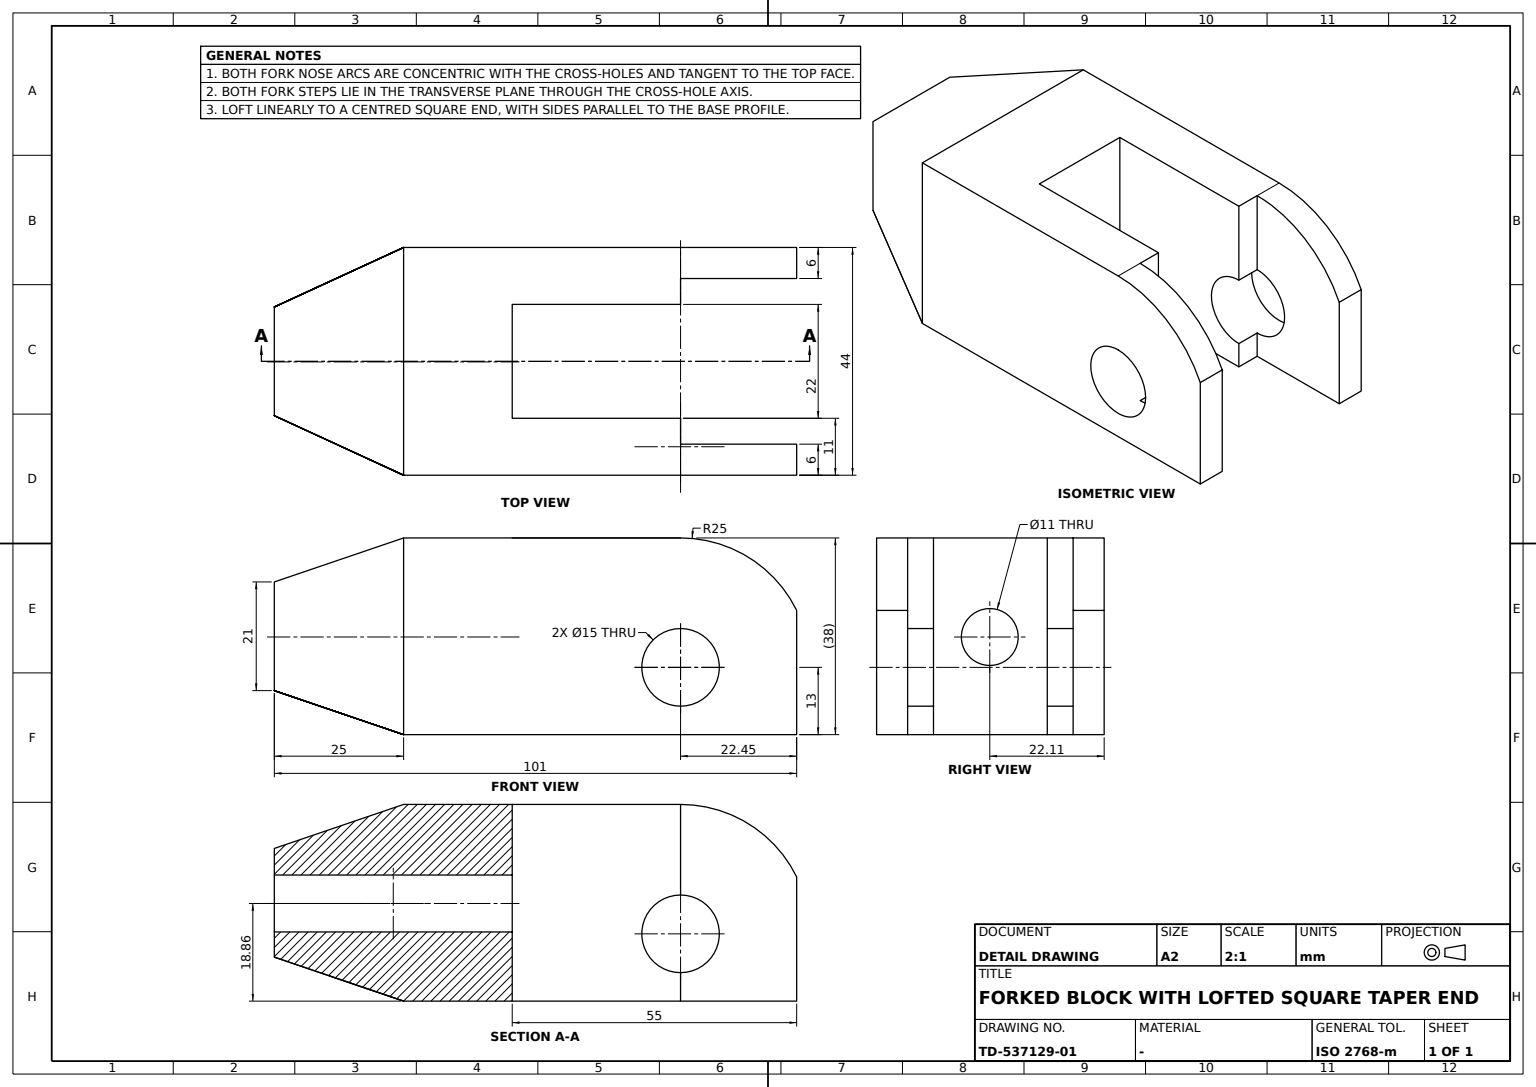
ISO-10303-21;
HEADER;
FILE_DESCRIPTION((''),'2;1');
FILE_NAME('','',(''),(''),'','','');
FILE_SCHEMA(('AUTOMOTIVE_DESIGN'));
ENDSEC;
DATA;
#1=APPLICATION_CONTEXT('');
#2=PRODUCT_CONTEXT('',#1,'mechanical');
#3=PRODUCT('','','',(#2));
#4=PRODUCT_DEFINITION_FORMATION('','',#3);
#5=PRODUCT_DEFINITION_CONTEXT('',#1,'design');
#6=PRODUCT_DEFINITION('','',#4,#5);
#7=PRODUCT_DEFINITION_SHAPE('','',#6);
#8=(LENGTH_UNIT()NAMED_UNIT(*)SI_UNIT(.MILLI.,.METRE.));
#9=(NAMED_UNIT(*)PLANE_ANGLE_UNIT()SI_UNIT($,.RADIAN.));
#10=(NAMED_UNIT(*)SI_UNIT($,.STERADIAN.)SOLID_ANGLE_UNIT());
#11=UNCERTAINTY_MEASURE_WITH_UNIT(LENGTH_MEASURE(1.E-05),#8,'distance_accuracy_value','');
#12=(GEOMETRIC_REPRESENTATION_CONTEXT(3)GLOBAL_UNCERTAINTY_ASSIGNED_CONTEXT((#11))GLOBAL_UNIT_ASSIGNED_CONTEXT((#8,#9,#10))REPRESENTATION_CONTEXT('',''));
#13=CARTESIAN_POINT('',(22.449944,16.,5.5));
#14=VERTEX_POINT('',#13);
#15=CARTESIAN_POINT('',(22.449944,22.,5.5));
#16=VERTEX_POINT('',#15);
#17=CARTESIAN_POINT('',(22.449944,-22.,5.5));
#18=DIRECTION('',(0.,1.,0.));
#19=VECTOR('',#18,1000.);
#20=LINE('',#17,#19);
#21=EDGE_CURVE('',#14,#16,#20,.T.);
#22=ORIENTED_EDGE('',*,*,#21,.T.);
#23=CARTESIAN_POINT('',(22.449944,22.,20.5));
#24=VERTEX_POINT('',#23);
#25=CARTESIAN_POINT('',(22.449944,22.,13.));
#26=DIRECTION('',(0.,-1.,0.));
#27=DIRECTION('',(1.,0.,0.));
#28=AXIS2_PLACEMENT_3D('',#25,#26,#27);
#29=CIRCLE('',#28,7.5);
#30=EDGE_CURVE('',#24,#16,#29,.T.);
#31=ORIENTED_EDGE('',*,*,#30,.F.);
#32=CARTESIAN_POINT('',(22.449944,16.,20.5));
#33=VERTEX_POINT('',#32);
#34=CARTESIAN_POINT('',(22.449944,-22.,20.5));
#35=LINE('',#34,#19);
#36=EDGE_CURVE('',#33,#24,#35,.T.);
#37=ORIENTED_EDGE('',*,*,#36,.F.);
#38=CARTESIAN_POINT('',(22.449944,16.,13.));
#39=DIRECTION('',(0.,0.,-1.));
#40=AXIS2_PLACEMENT_3D('',#38,#26,#39);
#41=CIRCLE('',#40,7.5);
#42=EDGE_CURVE('',#33,#14,#41,.T.);
#43=ORIENTED_EDGE('',*,*,#42,.T.);
#44=EDGE_LOOP('',(#22,#31,#37,#43));
#45=FACE_OUTER_BOUND('',#44,.T.);
#46=CARTESIAN_POINT('',(22.449944,-22.,13.));
#47=DIRECTION('',(0.,0.,1.));
#48=AXIS2_PLACEMENT_3D('',#46,#18,#47);
#49=CYLINDRICAL_SURFACE('',#48,7.5);
#50=ADVANCED_FACE('',(#45),#49,.F.);
#51=CARTESIAN_POINT('',(101.,10.495948,8.504359));
#52=VERTEX_POINT('',#51);
#53=CARTESIAN_POINT('',(76.,21.993633,0.005916));
#54=VERTEX_POINT('',#53);
#55=CARTESIAN_POINT('',(92.666667,14.327802,5.672203));
#56=CARTESIAN_POINT('',(84.333333,18.159656,2.840046));
#57=B_SPLINE_CURVE_WITH_KNOTS('',3,(#51,#55,#56,#53),.UNSPECIFIED.,.F.,.F.,(4,4),(0.,1.),.UNSPECIFIED.);
#58=EDGE_CURVE('',#52,#54,#57,.T.);
#59=ORIENTED_EDGE('',*,*,#58,.T.);
#60=CARTESIAN_POINT('',(76.,21.998212,2.362252));
#61=VERTEX_POINT('',#60);
#62=CARTESIAN_POINT('',(76.,22.005328,0.020728));
#63=CARTESIAN_POINT('',(76.,21.997336,0.079513));
#64=CARTESIAN_POINT('',(76.,22.001332,0.178516));
#65=CARTESIAN_POINT('',(76.,21.999112,0.360332));
#66=CARTESIAN_POINT('',(76.,22.000592,0.718464));
#67=CARTESIAN_POINT('',(76.,21.999652,1.404027));
#68=CARTESIAN_POINT('',(76.,21.999859,1.985808));
#69=B_SPLINE_CURVE_WITH_KNOTS('',3,(#53,#62,#63,#64,#65,#66,#67,#68,#60),.UNSPECIFIED.,.F.,.F.,(4,1,1,1,1,1,4),(0.,0.000976562,0.001953125,0.00390625,0.0078125,0.015625,0.02994468),.UNSPECIFIED.);
#70=EDGE_CURVE('',#54,#61,#69,.T.);
#71=ORIENTED_EDGE('',*,*,#70,.T.);
#72=CARTESIAN_POINT('',(76.,21.992469,37.990831));
#73=VERTEX_POINT('',#72);
#74=CARTESIAN_POINT('',(76.,21.999974,2.396567));
#75=CARTESIAN_POINT('',(76.,22.000206,3.252405));
#76=CARTESIAN_POINT('',(76.,21.999825,5.752273));
#77=CARTESIAN_POINT('',(76.,22.000117,11.504111));
#78=CARTESIAN_POINT('',(76.,21.999961,19.721555));
#79=CARTESIAN_POINT('',(76.,22.,27.938819));
#80=CARTESIAN_POINT('',(76.,22.,33.690928));
#81=CARTESIAN_POINT('',(76.,22.,36.361551));
#82=CARTESIAN_POINT('',(76.,22.,37.491429));
#83=CARTESIAN_POINT('',(76.,22.,37.812418));
#84=CARTESIAN_POINT('',(76.,22.,37.940813));
#85=CARTESIAN_POINT('',(76.,22.002328,37.971865));
#86=CARTESIAN_POINT('',(76.,21.997745,37.986565));
#87=CARTESIAN_POINT('',(76.,21.993856,37.989071));
#88=B_SPLINE_CURVE_WITH_KNOTS('',3,(#60,#74,#75,#76,#77,#78,#79,#80,#81,#82,#83,#84,#85,#86,#87,#72),.UNSPECIFIED.,.F.,.F.,(4,1,1,1,1,1,1,1,1,1,1,1,1,4),(0.02994468,0.03125,0.0625,0.125,0.25,0.375,0.4375,0.46875,0.4765625,0.48046875,0.480957031,0.481445312,0.481567383,0.481678034),.UNSPECIFIED.);
#89=EDGE_CURVE('',#61,#73,#88,.T.);
#90=ORIENTED_EDGE('',*,*,#89,.T.);
#91=CARTESIAN_POINT('',(76.,-22.,38.));
#92=VERTEX_POINT('',#91);
#93=CARTESIAN_POINT('',(76.,-7.333333,38.));
#94=CARTESIAN_POINT('',(76.,7.333333,38.));
#95=B_SPLINE_CURVE_WITH_KNOTS('',3,(#91,#93,#94,#72),.UNSPECIFIED.,.F.,.F.,(4,4),(0.,1.),.UNSPECIFIED.);
#96=EDGE_CURVE('',#92,#73,#95,.T.);
#97=ORIENTED_EDGE('',*,*,#96,.F.);
#98=CARTESIAN_POINT('',(101.,-10.5,29.5));
#99=VERTEX_POINT('',#98);
#100=CARTESIAN_POINT('',(84.333333,-18.166667,35.166667));
#101=CARTESIAN_POINT('',(92.666667,-14.333333,32.333333));
#102=B_SPLINE_CURVE_WITH_KNOTS('',3,(#91,#100,#101,#98),.UNSPECIFIED.,.F.,.F.,(4,4),(0.,1.),.UNSPECIFIED.);
#103=EDGE_CURVE('',#92,#99,#102,.T.);
#104=ORIENTED_EDGE('',*,*,#103,.T.);
#105=CARTESIAN_POINT('',(101.,10.502543,8.511455));
#106=CARTESIAN_POINT('',(101.,10.498729,8.543941));
#107=CARTESIAN_POINT('',(101.,10.500636,8.598653));
#108=CARTESIAN_POINT('',(101.,10.499576,8.699131));
#109=CARTESIAN_POINT('',(101.,10.500283,8.897046));
#110=CARTESIAN_POINT('',(101.,10.499812,9.294902));
#111=CARTESIAN_POINT('',(101.,10.500126,10.089264));
#112=CARTESIAN_POINT('',(101.,10.499916,11.678888));
#113=CARTESIAN_POINT('',(101.,10.500056,14.857535));
#114=CARTESIAN_POINT('',(101.,10.501476,19.400362));
#115=CARTESIAN_POINT('',(101.,10.495516,23.935049));
#116=CARTESIAN_POINT('',(101.,10.506725,27.125907));
#117=CARTESIAN_POINT('',(101.,10.491593,28.585496));
#118=CARTESIAN_POINT('',(101.,10.506305,29.225732));
#119=CARTESIAN_POINT('',(101.,10.492664,29.388443));
#120=CARTESIAN_POINT('',(101.,10.503941,29.471531));
#121=CARTESIAN_POINT('',(101.,10.502736,29.4862));
#122=CARTESIAN_POINT('',(101.,10.498467,29.49225));
#123=CARTESIAN_POINT('',(101.,10.494805,29.495405));
#124=CARTESIAN_POINT('',(101.,10.486541,29.498931));
#125=CARTESIAN_POINT('',(101.,10.464878,29.500457));
#126=CARTESIAN_POINT('',(101.,10.432319,29.500903));
#127=CARTESIAN_POINT('',(101.,10.398751,29.500263));
#128=CARTESIAN_POINT('',(101.,10.278255,29.498336));
#129=CARTESIAN_POINT('',(101.,10.067183,29.498289));
#130=CARTESIAN_POINT('',(101.,9.023461,29.503487));
#131=CARTESIAN_POINT('',(101.,7.226471,29.5));
#132=CARTESIAN_POINT('',(101.,3.85,29.5));
#133=CARTESIAN_POINT('',(101.,-2.058824,29.5));
#134=CARTESIAN_POINT('',(101.,-7.123529,29.5));
#135=B_SPLINE_CURVE_WITH_KNOTS('',3,(#51,#105,#106,#107,#108,#109,#110,#111,#112,#113,#114,#115,#116,#117,#118,#119,#120,#121,#122,#123,#124,#125,#126,#127,#128,#129,#130,#131,#132,#133,#134,#98),.UNSPECIFIED.,.F.,.F.,(4,1,1,1,1,1,1,1,1,1,1,1,1,1,1,1,1,1,1,1,1,1,1,1,1,1,1,1,1,4),(0.,0.000976562,0.001953125,0.00390625,0.0078125,0.015625,0.03125,0.0625,0.125,0.25,0.375,0.4375,0.46875,0.4765625,0.48046875,0.480957031,0.481445312,0.481567383,0.481689453,0.481933594,0.482421875,0.483398438,0.484375,0.484863281,0.4921875,0.5,0.5625,0.625,0.75,1.),.UNSPECIFIED.);
#136=EDGE_CURVE('',#52,#99,#135,.T.);
#137=ORIENTED_EDGE('',*,*,#136,.F.);
#138=EDGE_LOOP('',(#59,#71,#90,#97,#104,#137));
#139=FACE_OUTER_BOUND('',#138,.T.);
#140=CARTESIAN_POINT('',(76.,21.991511,0.007889));
#141=CARTESIAN_POINT('',(92.666667,14.336805,5.681213));
#142=CARTESIAN_POINT('',(84.333333,18.171066,2.85097));
#143=CARTESIAN_POINT('',(92.666667,14.331598,5.722465));
#144=CARTESIAN_POINT('',(84.333333,18.164467,2.900989));
#145=CARTESIAN_POINT('',(92.666667,14.334201,5.791941));
#146=CARTESIAN_POINT('',(84.333333,18.167767,2.985228));
#147=CARTESIAN_POINT('',(92.666667,14.332755,5.919531));
#148=CARTESIAN_POINT('',(84.333333,18.165933,3.139932));
#149=CARTESIAN_POINT('',(92.666667,14.333719,6.170852));
#150=CARTESIAN_POINT('',(84.333333,18.167156,3.444658));
#151=CARTESIAN_POINT('',(92.666667,14.333076,6.676066));
#152=CARTESIAN_POINT('',(84.333333,18.166341,4.05723));
#153=CARTESIAN_POINT('',(76.,21.999605,1.438394));
#154=CARTESIAN_POINT('',(92.666667,14.333505,7.684779));
#155=CARTESIAN_POINT('',(84.333333,18.166884,5.280295));
#156=CARTESIAN_POINT('',(76.,22.000263,2.87581));
#157=CARTESIAN_POINT('',(92.666667,14.333219,9.703349));
#158=CARTESIAN_POINT('',(84.333333,18.166522,7.727811));
#159=CARTESIAN_POINT('',(92.666667,14.33341,13.739727));
#160=CARTESIAN_POINT('',(84.333333,18.166763,12.621919));
#161=CARTESIAN_POINT('',(92.666667,14.334304,19.507427));
#162=CARTESIAN_POINT('',(84.333333,18.167133,19.614491));
#163=CARTESIAN_POINT('',(92.666667,14.330344,25.269639));
#164=CARTESIAN_POINT('',(84.333333,18.165172,26.604229));
#165=CARTESIAN_POINT('',(92.666667,14.337817,29.314248));
#166=CARTESIAN_POINT('',(84.333333,18.168908,31.502588));
#167=CARTESIAN_POINT('',(92.666667,14.327729,31.177514));
#168=CARTESIAN_POINT('',(84.333333,18.163864,33.769532));
#169=CARTESIAN_POINT('',(92.666667,14.337537,31.980964));
#170=CARTESIAN_POINT('',(84.333333,18.168768,34.736197));
#171=CARTESIAN_POINT('',(92.666667,14.328443,32.196435));
#172=CARTESIAN_POINT('',(84.333333,18.164221,35.004426));
#173=CARTESIAN_POINT('',(92.666667,14.33596,32.294625));
#174=CARTESIAN_POINT('',(84.333333,18.16798,35.117719));
#175=CARTESIAN_POINT('',(92.666667,14.335933,32.314755));
#176=CARTESIAN_POINT('',(84.333333,18.169131,35.14331));
#177=CARTESIAN_POINT('',(92.666667,14.331535,32.323766));
#178=CARTESIAN_POINT('',(84.333333,18.164604,35.155282));
#179=CARTESIAN_POINT('',(76.,21.997672,37.986798));
#180=CARTESIAN_POINT('',(92.666667,14.326291,32.327545));
#181=CARTESIAN_POINT('',(84.333333,18.157778,35.159685));
#182=CARTESIAN_POINT('',(76.,21.989264,37.991825));
#183=CARTESIAN_POINT('',(92.666667,14.317459,32.334298));
#184=CARTESIAN_POINT('',(84.333333,18.148378,35.169664));
#185=CARTESIAN_POINT('',(76.,21.979296,38.005031));
#186=CARTESIAN_POINT('',(92.666667,14.284217,32.332825));
#187=CARTESIAN_POINT('',(84.333333,18.103556,35.165193));
#188=CARTESIAN_POINT('',(76.,21.922896,37.997561));
#189=CARTESIAN_POINT('',(92.666667,14.239395,32.333041));
#190=CARTESIAN_POINT('',(84.333333,18.046471,35.165179));
#191=CARTESIAN_POINT('',(76.,21.853546,37.997317));
#192=CARTESIAN_POINT('',(92.666667,14.19507,32.333621));
#193=CARTESIAN_POINT('',(84.333333,17.991389,35.166978));
#194=CARTESIAN_POINT('',(76.,21.787708,38.000335));
#195=CARTESIAN_POINT('',(92.666667,14.031715,32.332224));
#196=CARTESIAN_POINT('',(84.333333,17.785174,35.166112));
#197=CARTESIAN_POINT('',(76.,21.538634,38.));
#198=CARTESIAN_POINT('',(92.666667,13.743614,32.332193));
#199=CARTESIAN_POINT('',(84.333333,17.420045,35.166096));
#200=CARTESIAN_POINT('',(76.,21.096477,38.));
#201=CARTESIAN_POINT('',(92.666667,12.315477,32.335658));
#202=CARTESIAN_POINT('',(84.333333,15.607494,35.167829));
#203=CARTESIAN_POINT('',(76.,18.89951,38.));
#204=CARTESIAN_POINT('',(92.666667,9.864706,32.333333));
#205=CARTESIAN_POINT('',(84.333333,12.502941,35.166667));
#206=CARTESIAN_POINT('',(76.,15.141176,38.));
#207=CARTESIAN_POINT('',(92.666667,5.255556,32.333333));
#208=CARTESIAN_POINT('',(84.333333,6.661111,35.166667));
#209=CARTESIAN_POINT('',(76.,8.066667,38.));
#210=CARTESIAN_POINT('',(92.666667,-2.810458,32.333333));
#211=CARTESIAN_POINT('',(84.333333,-3.562092,35.166667));
#212=CARTESIAN_POINT('',(76.,-4.313725,38.));
#213=CARTESIAN_POINT('',(92.666667,-9.724183,32.333333));
#214=CARTESIAN_POINT('',(84.333333,-12.324837,35.166667));
#215=CARTESIAN_POINT('',(76.,-14.92549,38.));
#216=B_SPLINE_SURFACE_WITH_KNOTS('',3,3,((#51,#55,#56,#140),(#105,#141,#142,#62),(#106,#143,#144,#63),(#107,#145,#146,#64),(#108,#147,#148,#65),(#109,#149,#150,#66),(#110,#151,#152,#153),(#111,#154,#155,#156),(#112,#157,#158,#76),(#113,#159,#160,#77),(#114,#161,#162,#78),(#115,#163,#164,#79),(#116,#165,#166,#80),(#117,#167,#168,#81),(#118,#169,#170,#82),(#119,#171,#172,#83),(#120,#173,#174,#84),(#121,#175,#176,#85),(#122,#177,#178,#179),(#123,#180,#181,#182),(#124,#183,#184,#185),(#125,#186,#187,#188),(#126,#189,#190,#191),(#127,#192,#193,#194),(#128,#195,#196,#197),(#129,#198,#199,#200),(#130,#201,#202,#203),(#131,#204,#205,#206),(#132,#207,#208,#209),(#133,#210,#211,#212),(#134,#213,#214,#215),(#98,#101,#100,#91)),.UNSPECIFIED.,.F.,.F.,.F.,(4,1,1,1,1,1,1,1,1,1,1,1,1,1,1,1,1,1,1,1,1,1,1,1,1,1,1,1,1,4),(4,4),(0.,0.000976562,0.001953125,0.00390625,0.0078125,0.015625,0.03125,0.0625,0.125,0.25,0.375,0.4375,0.46875,0.4765625,0.48046875,0.480957031,0.481445312,0.481567383,0.481689453,0.481933594,0.482421875,0.483398438,0.484375,0.484863281,0.4921875,0.5,0.5625,0.625,0.75,1.),(0.,1.),.UNSPECIFIED.);
#217=ADVANCED_FACE('',(#139),#216,.F.);
#218=VERTEX_POINT('',#34);
#219=VERTEX_POINT('',#17);
#220=AXIS2_PLACEMENT_3D('',#46,#26,#27);
#221=CIRCLE('',#220,7.5);
#222=EDGE_CURVE('',#218,#219,#221,.T.);
#223=ORIENTED_EDGE('',*,*,#222,.T.);
#224=CARTESIAN_POINT('',(22.449944,-16.,5.5));
#225=VERTEX_POINT('',#224);
#226=EDGE_CURVE('',#219,#225,#20,.T.);
#227=ORIENTED_EDGE('',*,*,#226,.T.);
#228=CARTESIAN_POINT('',(22.449944,-16.,20.5));
#229=VERTEX_POINT('',#228);
#230=CARTESIAN_POINT('',(22.449944,-16.,13.));
#231=AXIS2_PLACEMENT_3D('',#230,#18,#47);
#232=CIRCLE('',#231,7.5);
#233=EDGE_CURVE('',#225,#229,#232,.T.);
#234=ORIENTED_EDGE('',*,*,#233,.T.);
#235=EDGE_CURVE('',#218,#229,#35,.T.);
#236=ORIENTED_EDGE('',*,*,#235,.F.);
#237=EDGE_LOOP('',(#223,#227,#234,#236));
#238=FACE_OUTER_BOUND('',#237,.T.);
#239=ADVANCED_FACE('',(#238),#49,.F.);
#240=ORIENTED_EDGE('',*,*,#21,.F.);
#241=CARTESIAN_POINT('',(22.449944,11.,5.5));
#242=VERTEX_POINT('',#241);
#243=VECTOR('',#26,1000.);
#244=LINE('',#17,#243);
#245=EDGE_CURVE('',#14,#242,#244,.T.);
#246=ORIENTED_EDGE('',*,*,#245,.T.);
#247=CARTESIAN_POINT('',(22.449944,11.,20.5));
#248=VERTEX_POINT('',#247);
#249=CARTESIAN_POINT('',(22.449944,11.,13.));
#250=AXIS2_PLACEMENT_3D('',#249,#26,#39);
#251=CIRCLE('',#250,7.5);
#252=EDGE_CURVE('',#242,#248,#251,.T.);
#253=ORIENTED_EDGE('',*,*,#252,.T.);
#254=EDGE_CURVE('',#248,#33,#35,.T.);
#255=ORIENTED_EDGE('',*,*,#254,.T.);
#256=ORIENTED_EDGE('',*,*,#36,.T.);
#257=EDGE_CURVE('',#16,#24,#29,.T.);
#258=ORIENTED_EDGE('',*,*,#257,.F.);
#259=EDGE_LOOP('',(#240,#246,#253,#255,#256,#258));
#260=FACE_OUTER_BOUND('',#259,.T.);
#261=ADVANCED_FACE('',(#260),#49,.F.);
#262=CARTESIAN_POINT('',(22.449944,16.,38.));
#263=VERTEX_POINT('',#262);
#264=CARTESIAN_POINT('',(22.449944,16.,44.));
#265=VECTOR('',#47,1000.);
#266=LINE('',#264,#265);
#267=EDGE_CURVE('',#33,#263,#266,.T.);
#268=ORIENTED_EDGE('',*,*,#267,.F.);
#269=ORIENTED_EDGE('',*,*,#254,.F.);
#270=CARTESIAN_POINT('',(22.449944,11.,38.));
#271=VERTEX_POINT('',#270);
#272=CARTESIAN_POINT('',(22.449944,11.,44.));
#273=LINE('',#272,#265);
#274=EDGE_CURVE('',#248,#271,#273,.T.);
#275=ORIENTED_EDGE('',*,*,#274,.T.);
#276=CARTESIAN_POINT('',(22.449944,-22.,38.));
#277=LINE('',#276,#19);
#278=EDGE_CURVE('',#271,#263,#277,.T.);
#279=ORIENTED_EDGE('',*,*,#278,.T.);
#280=EDGE_LOOP('',(#268,#269,#275,#279));
#281=FACE_OUTER_BOUND('',#280,.T.);
#282=DIRECTION('',(-1.,0.,0.));
#283=AXIS2_PLACEMENT_3D('',#272,#282,#47);
#284=PLANE('',#283);
#285=ADVANCED_FACE('',(#281),#284,.T.);
#286=VERTEX_POINT('',#276);
#287=CARTESIAN_POINT('',(0.,-22.,24.));
#288=VERTEX_POINT('',#287);
#289=CIRCLE('',#220,25.);
#290=EDGE_CURVE('',#286,#288,#289,.T.);
#291=ORIENTED_EDGE('',*,*,#290,.F.);
#292=CARTESIAN_POINT('',(22.449944,-16.,38.));
#293=VERTEX_POINT('',#292);
#294=EDGE_CURVE('',#286,#293,#277,.T.);
#295=ORIENTED_EDGE('',*,*,#294,.T.);
#296=CARTESIAN_POINT('',(0.,-16.,24.));
#297=VERTEX_POINT('',#296);
#298=CIRCLE('',#231,25.);
#299=EDGE_CURVE('',#297,#293,#298,.T.);
#300=ORIENTED_EDGE('',*,*,#299,.F.);
#301=LINE('',#287,#19);
#302=EDGE_CURVE('',#288,#297,#301,.T.);
#303=ORIENTED_EDGE('',*,*,#302,.F.);
#304=EDGE_LOOP('',(#291,#295,#300,#303));
#305=FACE_OUTER_BOUND('',#304,.T.);
#306=CYLINDRICAL_SURFACE('',#48,25.);
#307=ADVANCED_FACE('',(#305),#306,.T.);
#308=CARTESIAN_POINT('',(76.,21.327697,0.));
#309=VERTEX_POINT('',#308);
#310=CARTESIAN_POINT('',(76.,21.773069,0.));
#311=CARTESIAN_POINT('',(76.,21.550383,0.));
#312=B_SPLINE_CURVE_WITH_KNOTS('',3,(#53,#310,#311,#308),.UNSPECIFIED.,.F.,.F.,(4,4),(0.,1.),.UNSPECIFIED.);
#313=EDGE_CURVE('',#54,#309,#312,.T.);
#314=ORIENTED_EDGE('',*,*,#313,.T.);
#315=CARTESIAN_POINT('',(76.,20.65519,0.));
#316=VERTEX_POINT('',#315);
#317=CARTESIAN_POINT('',(76.,21.103528,0.));
#318=CARTESIAN_POINT('',(76.,20.879359,0.));
#319=B_SPLINE_CURVE_WITH_KNOTS('',3,(#308,#317,#318,#315),.UNSPECIFIED.,.F.,.F.,(4,4),(0.,1.),.UNSPECIFIED.);
#320=EDGE_CURVE('',#309,#316,#319,.T.);
#321=ORIENTED_EDGE('',*,*,#320,.T.);
#322=CARTESIAN_POINT('',(76.,19.30979,0.));
#323=VERTEX_POINT('',#322);
#324=CARTESIAN_POINT('',(76.,20.206723,0.));
#325=CARTESIAN_POINT('',(76.,19.758256,0.));
#326=B_SPLINE_CURVE_WITH_KNOTS('',3,(#315,#324,#325,#322),.UNSPECIFIED.,.F.,.F.,(4,4),(0.,1.),.UNSPECIFIED.);
#327=EDGE_CURVE('',#316,#323,#326,.T.);
#328=ORIENTED_EDGE('',*,*,#327,.T.);
#329=CARTESIAN_POINT('',(76.,16.614761,0.));
#330=VERTEX_POINT('',#329);
#331=CARTESIAN_POINT('',(76.,18.411447,0.));
#332=CARTESIAN_POINT('',(76.,17.513104,0.));
#333=B_SPLINE_CURVE_WITH_KNOTS('',3,(#322,#331,#332,#329),.UNSPECIFIED.,.F.,.F.,(4,4),(0.,1.),.UNSPECIFIED.);
#334=EDGE_CURVE('',#323,#330,#333,.T.);
#335=ORIENTED_EDGE('',*,*,#334,.T.);
#336=CARTESIAN_POINT('',(76.,11.218305,0.));
#337=VERTEX_POINT('',#336);
#338=CARTESIAN_POINT('',(76.,14.815943,0.));
#339=CARTESIAN_POINT('',(76.,13.017124,0.));
#340=B_SPLINE_CURVE_WITH_KNOTS('',3,(#329,#338,#339,#336),.UNSPECIFIED.,.F.,.F.,(4,4),(0.,1.),.UNSPECIFIED.);
#341=EDGE_CURVE('',#330,#337,#340,.T.);
#342=ORIENTED_EDGE('',*,*,#341,.T.);
#343=CARTESIAN_POINT('',(76.,-0.120378,0.));
#344=VERTEX_POINT('',#343);
#345=CARTESIAN_POINT('',(76.,7.438744,0.));
#346=CARTESIAN_POINT('',(76.,3.659183,0.));
#347=B_SPLINE_CURVE_WITH_KNOTS('',3,(#336,#345,#346,#343),.UNSPECIFIED.,.F.,.F.,(4,4),(0.,1.),.UNSPECIFIED.);
#348=EDGE_CURVE('',#337,#344,#347,.T.);
#349=ORIENTED_EDGE('',*,*,#348,.T.);
#350=CARTESIAN_POINT('',(76.,-17.491021,0.));
#351=VERTEX_POINT('',#350);
#352=CARTESIAN_POINT('',(76.,-5.910593,0.));
#353=CARTESIAN_POINT('',(76.,-11.700807,0.));
#354=B_SPLINE_CURVE_WITH_KNOTS('',3,(#343,#352,#353,#350),.UNSPECIFIED.,.F.,.F.,(4,4),(0.,1.),.UNSPECIFIED.);
#355=EDGE_CURVE('',#344,#351,#354,.T.);
#356=ORIENTED_EDGE('',*,*,#355,.T.);
#357=CARTESIAN_POINT('',(76.,-21.780355,0.));
#358=VERTEX_POINT('',#357);
#359=CARTESIAN_POINT('',(76.,-18.920799,0.));
#360=CARTESIAN_POINT('',(76.,-20.350577,0.));
#361=B_SPLINE_CURVE_WITH_KNOTS('',3,(#350,#359,#360,#357),.UNSPECIFIED.,.F.,.F.,(4,4),(0.,1.),.UNSPECIFIED.);
#362=EDGE_CURVE('',#351,#358,#361,.T.);
#363=ORIENTED_EDGE('',*,*,#362,.T.);
#364=CARTESIAN_POINT('',(76.,-21.935414,0.));
#365=VERTEX_POINT('',#364);
#366=CARTESIAN_POINT('',(76.,-21.832041,0.));
#367=CARTESIAN_POINT('',(76.,-21.883727,0.));
#368=B_SPLINE_CURVE_WITH_KNOTS('',3,(#357,#366,#367,#364),.UNSPECIFIED.,.F.,.F.,(4,4),(0.,1.),.UNSPECIFIED.);
#369=EDGE_CURVE('',#358,#365,#368,.T.);
#370=ORIENTED_EDGE('',*,*,#369,.T.);
#371=CARTESIAN_POINT('',(76.,-21.979602,0.));
#372=VERTEX_POINT('',#371);
#373=CARTESIAN_POINT('',(76.,-21.950143,0.));
#374=CARTESIAN_POINT('',(76.,-21.964873,0.));
#375=B_SPLINE_CURVE_WITH_KNOTS('',3,(#364,#373,#374,#371),.UNSPECIFIED.,.F.,.F.,(4,4),(0.,1.),.UNSPECIFIED.);
#376=EDGE_CURVE('',#365,#372,#375,.T.);
#377=ORIENTED_EDGE('',*,*,#376,.T.);
#378=CARTESIAN_POINT('',(76.,-22.,0.));
#379=VERTEX_POINT('',#378);
#380=LINE('',#378,#19);
#381=EDGE_CURVE('',#379,#372,#380,.T.);
#382=ORIENTED_EDGE('',*,*,#381,.F.);
#383=CARTESIAN_POINT('',(0.,-22.,0.));
#384=VERTEX_POINT('',#383);
#385=VECTOR('',#27,1000.);
#386=LINE('',#383,#385);
#387=EDGE_CURVE('',#384,#379,#386,.T.);
#388=ORIENTED_EDGE('',*,*,#387,.F.);
#389=CARTESIAN_POINT('',(0.,-16.,0.));
#390=VERTEX_POINT('',#389);
#391=LINE('',#383,#19);
#392=EDGE_CURVE('',#384,#390,#391,.T.);
#393=ORIENTED_EDGE('',*,*,#392,.T.);
#394=CARTESIAN_POINT('',(22.449944,-16.,0.));
#395=VERTEX_POINT('',#394);
#396=LINE('',#389,#385);
#397=EDGE_CURVE('',#390,#395,#396,.T.);
#398=ORIENTED_EDGE('',*,*,#397,.T.);
#399=CARTESIAN_POINT('',(22.449944,-11.,0.));
#400=VERTEX_POINT('',#399);
#401=LINE('',#394,#19);
#402=EDGE_CURVE('',#395,#400,#401,.T.);
#403=ORIENTED_EDGE('',*,*,#402,.T.);
#404=CARTESIAN_POINT('',(55.,-11.,0.));
#405=VERTEX_POINT('',#404);
#406=LINE('',#399,#385);
#407=EDGE_CURVE('',#400,#405,#406,.T.);
#408=ORIENTED_EDGE('',*,*,#407,.T.);
#409=CARTESIAN_POINT('',(55.,11.,0.));
#410=VERTEX_POINT('',#409);
#411=CARTESIAN_POINT('',(55.,0.,0.));
#412=LINE('',#411,#19);
#413=EDGE_CURVE('',#405,#410,#412,.T.);
#414=ORIENTED_EDGE('',*,*,#413,.T.);
#415=CARTESIAN_POINT('',(22.449944,11.,0.));
#416=VERTEX_POINT('',#415);
#417=VECTOR('',#282,1000.);
#418=LINE('',#409,#417);
#419=EDGE_CURVE('',#410,#416,#418,.T.);
#420=ORIENTED_EDGE('',*,*,#419,.T.);
#421=CARTESIAN_POINT('',(22.449944,16.,0.));
#422=VERTEX_POINT('',#421);
#423=LINE('',#415,#19);
#424=EDGE_CURVE('',#416,#422,#423,.T.);
#425=ORIENTED_EDGE('',*,*,#424,.T.);
#426=CARTESIAN_POINT('',(0.,16.,0.));
#427=VERTEX_POINT('',#426);
#428=LINE('',#421,#417);
#429=EDGE_CURVE('',#422,#427,#428,.T.);
#430=ORIENTED_EDGE('',*,*,#429,.T.);
#431=CARTESIAN_POINT('',(0.,22.,0.));
#432=VERTEX_POINT('',#431);
#433=EDGE_CURVE('',#427,#432,#391,.T.);
#434=ORIENTED_EDGE('',*,*,#433,.T.);
#435=CARTESIAN_POINT('',(1.095788,22.,0.));
#436=LINE('',#435,#385);
#437=EDGE_CURVE('',#432,#54,#436,.T.);
#438=ORIENTED_EDGE('',*,*,#437,.T.);
#439=EDGE_LOOP('',(#314,#321,#328,#335,#342,#349,#356,#363,#370,#377,#382,#388,#393,#398,#403,#408,#414,#420,#425,#430,#434,#438));
#440=FACE_OUTER_BOUND('',#439,.T.);
#441=CARTESIAN_POINT('',(1.095788,-22.,0.));
#442=AXIS2_PLACEMENT_3D('',#441,#47,#27);
#443=PLANE('',#442);
#444=ADVANCED_FACE('',(#440),#443,.F.);
#445=ORIENTED_EDGE('',*,*,#376,.F.);
#446=ORIENTED_EDGE('',*,*,#369,.F.);
#447=ORIENTED_EDGE('',*,*,#362,.F.);
#448=ORIENTED_EDGE('',*,*,#355,.F.);
#449=ORIENTED_EDGE('',*,*,#348,.F.);
#450=ORIENTED_EDGE('',*,*,#341,.F.);
#451=ORIENTED_EDGE('',*,*,#334,.F.);
#452=ORIENTED_EDGE('',*,*,#327,.F.);
#453=ORIENTED_EDGE('',*,*,#320,.F.);
#454=ORIENTED_EDGE('',*,*,#313,.F.);
#455=ORIENTED_EDGE('',*,*,#58,.F.);
#456=CARTESIAN_POINT('',(101.,-10.5,25.867089));
#457=CARTESIAN_POINT('',(101.,-10.502989,20.414505));
#458=CARTESIAN_POINT('',(101.,-10.495516,14.064951));
#459=CARTESIAN_POINT('',(101.,-10.506725,10.874093));
#460=CARTESIAN_POINT('',(101.,-10.491593,9.414504));
#461=CARTESIAN_POINT('',(101.,-10.506305,8.774268));
#462=CARTESIAN_POINT('',(101.,-10.492664,8.611557));
#463=CARTESIAN_POINT('',(101.,-10.503941,8.528469));
#464=CARTESIAN_POINT('',(101.,-10.502736,8.5138));
#465=CARTESIAN_POINT('',(101.,-10.498467,8.50775));
#466=CARTESIAN_POINT('',(101.,-10.494805,8.504595));
#467=CARTESIAN_POINT('',(101.,-10.486541,8.501069));
#468=CARTESIAN_POINT('',(101.,-10.464878,8.499543));
#469=CARTESIAN_POINT('',(101.,-10.432319,8.499097));
#470=CARTESIAN_POINT('',(101.,-10.398751,8.499737));
#471=CARTESIAN_POINT('',(101.,-10.278255,8.501664));
#472=CARTESIAN_POINT('',(101.,-10.067186,8.501707));
#473=CARTESIAN_POINT('',(101.,-9.4439,8.498257));
#474=CARTESIAN_POINT('',(101.,-8.492648,8.500001));
#475=CARTESIAN_POINT('',(101.,-6.804416,8.500005));
#476=CARTESIAN_POINT('',(101.,-3.850012,8.500013));
#477=CARTESIAN_POINT('',(101.,0.370578,8.500011));
#478=CARTESIAN_POINT('',(101.,4.591232,8.49994));
#479=CARTESIAN_POINT('',(101.,7.545505,8.50009));
#480=CARTESIAN_POINT('',(101.,9.02292,8.499865));
#481=CARTESIAN_POINT('',(101.,9.761209,8.500203));
#482=CARTESIAN_POINT('',(101.,10.130981,8.499696));
#483=CARTESIAN_POINT('',(101.,10.314925,8.500456));
#484=CARTESIAN_POINT('',(101.,10.40831,8.499316));
#485=CARTESIAN_POINT('',(101.,10.459161,8.501368));
#486=CARTESIAN_POINT('',(101.,10.489354,8.497264));
#487=B_SPLINE_CURVE_WITH_KNOTS('',3,(#98,#456,#457,#458,#459,#460,#461,#462,#463,#464,#465,#466,#467,#468,#469,#470,#471,#472,#473,#474,#475,#476,#477,#478,#479,#480,#481,#482,#483,#484,#485,#486,#51),.UNSPECIFIED.,.F.,.F.,(4,1,1,1,1,1,1,1,1,1,1,1,1,1,1,1,1,1,1,1,1,1,1,1,1,1,1,1,1,1,4),(0.,0.25,0.375,0.4375,0.46875,0.4765625,0.48046875,0.480957031,0.481445312,0.481567383,0.481689453,0.481933594,0.482421875,0.483398438,0.484375,0.484863281,0.4921875,0.5,0.53125,0.5625,0.625,0.75,0.875,0.9375,0.96875,0.984375,0.9921875,0.99609375,0.998046875,0.999023438,1.),.UNSPECIFIED.);
#488=EDGE_CURVE('',#99,#52,#487,.T.);
#489=ORIENTED_EDGE('',*,*,#488,.F.);
#490=ORIENTED_EDGE('',*,*,#103,.F.);
#491=CARTESIAN_POINT('',(76.,-21.979876,0.000113));
#492=CARTESIAN_POINT('',(76.,-21.984829,0.002299));
#493=CARTESIAN_POINT('',(76.,-21.989264,0.008175));
#494=CARTESIAN_POINT('',(76.,-21.997672,0.013202));
#495=CARTESIAN_POINT('',(76.,-22.002328,0.028135));
#496=CARTESIAN_POINT('',(76.,-22.,0.059187));
#497=CARTESIAN_POINT('',(76.,-22.,0.187582));
#498=CARTESIAN_POINT('',(76.,-22.,0.508571));
#499=CARTESIAN_POINT('',(76.,-22.,1.638449));
#500=CARTESIAN_POINT('',(76.,-22.,4.309072));
#501=CARTESIAN_POINT('',(76.,-22.,10.061181));
#502=CARTESIAN_POINT('',(76.,-22.,21.565401));
#503=CARTESIAN_POINT('',(76.,-22.,31.42616));
#504=B_SPLINE_CURVE_WITH_KNOTS('',3,(#371,#491,#492,#493,#494,#495,#496,#497,#498,#499,#500,#501,#502,#503,#91),.UNSPECIFIED.,.F.,.F.,(4,1,1,1,1,1,1,1,1,1,1,1,4),(0.518052409,0.518066406,0.518310547,0.518432617,0.518554688,0.519042969,0.51953125,0.5234375,0.53125,0.5625,0.625,0.75,1.),.UNSPECIFIED.);
#505=EDGE_CURVE('',#372,#92,#504,.T.);
#506=ORIENTED_EDGE('',*,*,#505,.F.);
#507=EDGE_LOOP('',(#445,#446,#447,#448,#449,#450,#451,#452,#453,#454,#455,#489,#490,#506));
#508=FACE_OUTER_BOUND('',#507,.T.);
#509=CARTESIAN_POINT('',(92.666667,-14.333333,27.720113));
#510=CARTESIAN_POINT('',(84.333333,-18.166667,29.573136));
#511=CARTESIAN_POINT('',(92.666667,-14.335326,20.798137));
#512=CARTESIAN_POINT('',(84.333333,-18.167663,21.181769));
#513=CARTESIAN_POINT('',(92.666667,-14.330344,12.730361));
#514=CARTESIAN_POINT('',(84.333333,-18.165172,11.395771));
#515=CARTESIAN_POINT('',(92.666667,-14.337817,8.685752));
#516=CARTESIAN_POINT('',(84.333333,-18.168908,6.497412));
#517=CARTESIAN_POINT('',(92.666667,-14.327729,6.822486));
#518=CARTESIAN_POINT('',(84.333333,-18.163864,4.230468));
#519=CARTESIAN_POINT('',(92.666667,-14.337537,6.019036));
#520=CARTESIAN_POINT('',(84.333333,-18.168768,3.263803));
#521=CARTESIAN_POINT('',(92.666667,-14.328443,5.803565));
#522=CARTESIAN_POINT('',(84.333333,-18.164221,2.995574));
#523=CARTESIAN_POINT('',(92.666667,-14.33596,5.705375));
#524=CARTESIAN_POINT('',(84.333333,-18.16798,2.882281));
#525=CARTESIAN_POINT('',(92.666667,-14.335933,5.685245));
#526=CARTESIAN_POINT('',(84.333333,-18.169131,2.85669));
#527=CARTESIAN_POINT('',(92.666667,-14.331535,5.676234));
#528=CARTESIAN_POINT('',(84.333333,-18.164604,2.844718));
#529=CARTESIAN_POINT('',(92.666667,-14.326291,5.672455));
#530=CARTESIAN_POINT('',(84.333333,-18.157778,2.840315));
#531=CARTESIAN_POINT('',(92.666667,-14.317459,5.665702));
#532=CARTESIAN_POINT('',(84.333333,-18.148378,2.830336));
#533=CARTESIAN_POINT('',(76.,-21.979296,-0.005031));
#534=CARTESIAN_POINT('',(92.666667,-14.284217,5.667175));
#535=CARTESIAN_POINT('',(84.333333,-18.103556,2.834807));
#536=CARTESIAN_POINT('',(76.,-21.922896,0.002439));
#537=CARTESIAN_POINT('',(92.666667,-14.239395,5.666959));
#538=CARTESIAN_POINT('',(84.333333,-18.046471,2.834821));
#539=CARTESIAN_POINT('',(76.,-21.853546,0.002683));
#540=CARTESIAN_POINT('',(92.666667,-14.19507,5.666379));
#541=CARTESIAN_POINT('',(84.333333,-17.991389,2.833022));
#542=CARTESIAN_POINT('',(76.,-21.787708,-0.000335));
#543=CARTESIAN_POINT('',(92.666667,-14.031715,5.667776));
#544=CARTESIAN_POINT('',(84.333333,-17.785174,2.833888));
#545=CARTESIAN_POINT('',(76.,-21.538634,0.));
#546=CARTESIAN_POINT('',(92.666667,-13.743616,5.667805));
#547=CARTESIAN_POINT('',(84.333333,-17.420047,2.833902));
#548=CARTESIAN_POINT('',(76.,-21.096477,0.));
#549=CARTESIAN_POINT('',(92.666667,-12.890541,5.665504));
#550=CARTESIAN_POINT('',(84.333333,-16.337182,2.832752));
#551=CARTESIAN_POINT('',(76.,-19.783823,0.));
#552=CARTESIAN_POINT('',(92.666667,-11.593138,5.666668));
#553=CARTESIAN_POINT('',(84.333333,-14.693629,2.833335));
#554=CARTESIAN_POINT('',(76.,-17.794119,0.000002));
#555=CARTESIAN_POINT('',(92.666667,-9.288568,5.666672));
#556=CARTESIAN_POINT('',(84.333333,-11.77272,2.83334));
#557=CARTESIAN_POINT('',(76.,-14.256872,0.000008));
#558=CARTESIAN_POINT('',(92.666667,-5.255572,5.666683));
#559=CARTESIAN_POINT('',(84.333333,-6.661132,2.833353));
#560=CARTESIAN_POINT('',(76.,-8.066692,0.000024));
#561=CARTESIAN_POINT('',(92.666667,0.505868,5.666681));
#562=CARTESIAN_POINT('',(84.333333,0.641158,2.833351));
#563=CARTESIAN_POINT('',(76.,0.776448,0.000021));
#564=CARTESIAN_POINT('',(92.666667,6.267396,5.66659));
#565=CARTESIAN_POINT('',(84.333333,7.943561,2.833241));
#566=CARTESIAN_POINT('',(76.,9.619725,-0.000109));
#567=CARTESIAN_POINT('',(92.666667,10.300213,5.666781));
#568=CARTESIAN_POINT('',(84.333333,13.054921,2.833472));
#569=CARTESIAN_POINT('',(76.,15.809629,0.000163));
#570=CARTESIAN_POINT('',(92.666667,12.317001,5.666495));
#571=CARTESIAN_POINT('',(84.333333,15.611083,2.833125));
#572=CARTESIAN_POINT('',(76.,18.905165,-0.000244));
#573=CARTESIAN_POINT('',(92.666667,13.324825,5.666924));
#574=CARTESIAN_POINT('',(84.333333,16.88844,2.833645));
#575=CARTESIAN_POINT('',(76.,20.452056,0.000367));
#576=CARTESIAN_POINT('',(92.666667,13.829593,5.666281));
#577=CARTESIAN_POINT('',(84.333333,17.528205,2.832865));
#578=CARTESIAN_POINT('',(76.,21.226817,-0.00055));
#579=CARTESIAN_POINT('',(92.666667,14.080692,5.667246));
#580=CARTESIAN_POINT('',(84.333333,17.846458,2.834035));
#581=CARTESIAN_POINT('',(76.,21.612225,0.000825));
#582=CARTESIAN_POINT('',(92.666667,14.20817,5.665798));
#583=CARTESIAN_POINT('',(84.333333,18.008029,2.83228));
#584=CARTESIAN_POINT('',(76.,21.807888,-0.001238));
#585=CARTESIAN_POINT('',(92.666667,14.277584,5.668404));
#586=CARTESIAN_POINT('',(84.333333,18.096008,2.83544));
#587=CARTESIAN_POINT('',(76.,21.914432,0.002475));
#588=CARTESIAN_POINT('',(92.666667,14.3188,5.663192));
#589=CARTESIAN_POINT('',(84.333333,18.148247,2.829121));
#590=CARTESIAN_POINT('',(76.,21.977693,-0.004951));
#591=B_SPLINE_SURFACE_WITH_KNOTS('',3,3,((#98,#101,#100,#91),(#456,#509,#510,#503),(#457,#511,#512,#502),(#458,#513,#514,#501),(#459,#515,#516,#500),(#460,#517,#518,#499),(#461,#519,#520,#498),(#462,#521,#522,#497),(#463,#523,#524,#496),(#464,#525,#526,#495),(#465,#527,#528,#494),(#466,#529,#530,#493),(#467,#531,#532,#533),(#468,#534,#535,#536),(#469,#537,#538,#539),(#470,#540,#541,#542),(#471,#543,#544,#545),(#472,#546,#547,#548),(#473,#549,#550,#551),(#474,#552,#553,#554),(#475,#555,#556,#557),(#476,#558,#559,#560),(#477,#561,#562,#563),(#478,#564,#565,#566),(#479,#567,#568,#569),(#480,#570,#571,#572),(#481,#573,#574,#575),(#482,#576,#577,#578),(#483,#579,#580,#581),(#484,#582,#583,#584),(#485,#585,#586,#587),(#486,#588,#589,#590),(#51,#55,#56,#140)),.UNSPECIFIED.,.F.,.F.,.F.,(4,1,1,1,1,1,1,1,1,1,1,1,1,1,1,1,1,1,1,1,1,1,1,1,1,1,1,1,1,1,4),(4,4),(0.,0.25,0.375,0.4375,0.46875,0.4765625,0.48046875,0.480957031,0.481445312,0.481567383,0.481689453,0.481933594,0.482421875,0.483398438,0.484375,0.484863281,0.4921875,0.5,0.53125,0.5625,0.625,0.75,0.875,0.9375,0.96875,0.984375,0.9921875,0.99609375,0.998046875,0.999023438,1.),(0.,1.),.UNSPECIFIED.);
#592=ADVANCED_FACE('',(#508),#591,.F.);
#593=ORIENTED_EDGE('',*,*,#30,.T.);
#594=ORIENTED_EDGE('',*,*,#257,.T.);
#595=EDGE_LOOP('',(#593,#594));
#596=FACE_BOUND('',#595,.T.);
#597=ORIENTED_EDGE('',*,*,#70,.F.);
#598=ORIENTED_EDGE('',*,*,#437,.F.);
#599=CARTESIAN_POINT('',(0.,22.,24.));
#600=VERTEX_POINT('',#599);
#601=VECTOR('',#39,1000.);
#602=LINE('',#599,#601);
#603=EDGE_CURVE('',#600,#432,#602,.T.);
#604=ORIENTED_EDGE('',*,*,#603,.F.);
#605=CARTESIAN_POINT('',(22.449944,22.,38.));
#606=VERTEX_POINT('',#605);
#607=CIRCLE('',#28,25.);
#608=EDGE_CURVE('',#606,#600,#607,.T.);
#609=ORIENTED_EDGE('',*,*,#608,.F.);
#610=CARTESIAN_POINT('',(76.,22.,38.));
#611=LINE('',#610,#417);
#612=EDGE_CURVE('',#73,#606,#611,.T.);
#613=ORIENTED_EDGE('',*,*,#612,.F.);
#614=ORIENTED_EDGE('',*,*,#89,.F.);
#615=EDGE_LOOP('',(#597,#598,#604,#609,#613,#614));
#616=FACE_OUTER_BOUND('',#615,.T.);
#617=AXIS2_PLACEMENT_3D('',#25,#26,#39);
#618=PLANE('',#617);
#619=ADVANCED_FACE('',(#596,#616),#618,.F.);
#620=CARTESIAN_POINT('',(22.449944,-11.,5.5));
#621=VERTEX_POINT('',#620);
#622=EDGE_CURVE('',#621,#225,#244,.T.);
#623=ORIENTED_EDGE('',*,*,#622,.T.);
#624=ORIENTED_EDGE('',*,*,#226,.F.);
#625=EDGE_CURVE('',#219,#218,#221,.T.);
#626=ORIENTED_EDGE('',*,*,#625,.T.);
#627=ORIENTED_EDGE('',*,*,#235,.T.);
#628=CARTESIAN_POINT('',(22.449944,-11.,20.5));
#629=VERTEX_POINT('',#628);
#630=EDGE_CURVE('',#229,#629,#35,.T.);
#631=ORIENTED_EDGE('',*,*,#630,.T.);
#632=CARTESIAN_POINT('',(22.449944,-11.,13.));
#633=AXIS2_PLACEMENT_3D('',#632,#18,#282);
#634=CIRCLE('',#633,7.5);
#635=EDGE_CURVE('',#629,#621,#634,.T.);
#636=ORIENTED_EDGE('',*,*,#635,.T.);
#637=EDGE_LOOP('',(#623,#624,#626,#627,#631,#636));
#638=FACE_OUTER_BOUND('',#637,.T.);
#639=ADVANCED_FACE('',(#638),#49,.F.);
#640=CARTESIAN_POINT('',(22.449944,-11.,38.));
#641=VERTEX_POINT('',#640);
#642=CARTESIAN_POINT('',(22.449944,-11.,44.));
#643=LINE('',#642,#265);
#644=EDGE_CURVE('',#629,#641,#643,.T.);
#645=ORIENTED_EDGE('',*,*,#644,.F.);
#646=ORIENTED_EDGE('',*,*,#630,.F.);
#647=CARTESIAN_POINT('',(22.449944,-16.,44.));
#648=LINE('',#647,#265);
#649=EDGE_CURVE('',#229,#293,#648,.T.);
#650=ORIENTED_EDGE('',*,*,#649,.T.);
#651=EDGE_CURVE('',#293,#641,#277,.T.);
#652=ORIENTED_EDGE('',*,*,#651,.T.);
#653=EDGE_LOOP('',(#645,#646,#650,#652));
#654=FACE_OUTER_BOUND('',#653,.T.);
#655=AXIS2_PLACEMENT_3D('',#647,#282,#26);
#656=PLANE('',#655);
#657=ADVANCED_FACE('',(#654),#656,.T.);
#658=CARTESIAN_POINT('',(55.,-11.,38.));
#659=VERTEX_POINT('',#658);
#660=CARTESIAN_POINT('',(55.,11.,38.));
#661=VERTEX_POINT('',#660);
#662=CARTESIAN_POINT('',(55.,-22.,38.));
#663=LINE('',#662,#19);
#664=EDGE_CURVE('',#659,#661,#663,.T.);
#665=ORIENTED_EDGE('',*,*,#664,.T.);
#666=CARTESIAN_POINT('',(55.,11.,44.));
#667=LINE('',#666,#265);
#668=EDGE_CURVE('',#410,#661,#667,.T.);
#669=ORIENTED_EDGE('',*,*,#668,.F.);
#670=ORIENTED_EDGE('',*,*,#413,.F.);
#671=CARTESIAN_POINT('',(55.,-11.,44.));
#672=LINE('',#671,#265);
#673=EDGE_CURVE('',#405,#659,#672,.T.);
#674=ORIENTED_EDGE('',*,*,#673,.T.);
#675=EDGE_LOOP('',(#665,#669,#670,#674));
#676=FACE_OUTER_BOUND('',#675,.T.);
#677=CARTESIAN_POINT('',(55.,0.114025,24.363698));
#678=VERTEX_POINT('',#677);
#679=CARTESIAN_POINT('',(55.,0.114025,13.363698));
#680=VERTEX_POINT('',#679);
#681=CARTESIAN_POINT('',(55.,0.114025,18.863698));
#682=AXIS2_PLACEMENT_3D('',#681,#282,#47);
#683=CIRCLE('',#682,5.5);
#684=EDGE_CURVE('',#678,#680,#683,.T.);
#685=ORIENTED_EDGE('',*,*,#684,.F.);
#686=EDGE_CURVE('',#680,#678,#683,.T.);
#687=ORIENTED_EDGE('',*,*,#686,.F.);
#688=EDGE_LOOP('',(#685,#687));
#689=FACE_BOUND('',#688,.T.);
#690=CARTESIAN_POINT('',(55.,0.,44.));
#691=AXIS2_PLACEMENT_3D('',#690,#282,#47);
#692=PLANE('',#691);
#693=ADVANCED_FACE('',(#676,#689),#692,.T.);
#694=EDGE_CURVE('',#395,#225,#648,.T.);
#695=ORIENTED_EDGE('',*,*,#694,.F.);
#696=ORIENTED_EDGE('',*,*,#397,.F.);
#697=CARTESIAN_POINT('',(0.,-16.,44.));
#698=LINE('',#697,#601);
#699=EDGE_CURVE('',#297,#390,#698,.T.);
#700=ORIENTED_EDGE('',*,*,#699,.F.);
#701=ORIENTED_EDGE('',*,*,#299,.T.);
#702=ORIENTED_EDGE('',*,*,#649,.F.);
#703=ORIENTED_EDGE('',*,*,#233,.F.);
#704=EDGE_LOOP('',(#695,#696,#700,#701,#702,#703));
#705=FACE_OUTER_BOUND('',#704,.T.);
#706=AXIS2_PLACEMENT_3D('',#697,#18,#47);
#707=PLANE('',#706);
#708=ADVANCED_FACE('',(#705),#707,.T.);
#709=ORIENTED_EDGE('',*,*,#278,.F.);
#710=CARTESIAN_POINT('',(76.,11.,38.));
#711=LINE('',#710,#417);
#712=EDGE_CURVE('',#661,#271,#711,.T.);
#713=ORIENTED_EDGE('',*,*,#712,.F.);
#714=ORIENTED_EDGE('',*,*,#664,.F.);
#715=CARTESIAN_POINT('',(76.,-11.,38.));
#716=LINE('',#715,#385);
#717=EDGE_CURVE('',#641,#659,#716,.T.);
#718=ORIENTED_EDGE('',*,*,#717,.F.);
#719=ORIENTED_EDGE('',*,*,#651,.F.);
#720=ORIENTED_EDGE('',*,*,#294,.F.);
#721=LINE('',#91,#417);
#722=EDGE_CURVE('',#92,#286,#721,.T.);
#723=ORIENTED_EDGE('',*,*,#722,.F.);
#724=ORIENTED_EDGE('',*,*,#96,.T.);
#725=ORIENTED_EDGE('',*,*,#612,.T.);
#726=EDGE_CURVE('',#263,#606,#277,.T.);
#727=ORIENTED_EDGE('',*,*,#726,.F.);
#728=EDGE_LOOP('',(#709,#713,#714,#718,#719,#720,#723,#724,#725,#727));
#729=FACE_OUTER_BOUND('',#728,.T.);
#730=AXIS2_PLACEMENT_3D('',#91,#39,#282);
#731=PLANE('',#730);
#732=ADVANCED_FACE('',(#729),#731,.F.);
#733=CARTESIAN_POINT('',(0.,16.,24.));
#734=VERTEX_POINT('',#733);
#735=CARTESIAN_POINT('',(0.,16.,44.));
#736=LINE('',#735,#601);
#737=EDGE_CURVE('',#734,#427,#736,.T.);
#738=ORIENTED_EDGE('',*,*,#737,.F.);
#739=EDGE_CURVE('',#734,#600,#301,.T.);
#740=ORIENTED_EDGE('',*,*,#739,.T.);
#741=ORIENTED_EDGE('',*,*,#603,.T.);
#742=ORIENTED_EDGE('',*,*,#433,.F.);
#743=EDGE_LOOP('',(#738,#740,#741,#742));
#744=FACE_OUTER_BOUND('',#743,.T.);
#745=AXIS2_PLACEMENT_3D('',#287,#27,#39);
#746=PLANE('',#745);
#747=ADVANCED_FACE('',(#744),#746,.F.);
#748=ORIENTED_EDGE('',*,*,#381,.T.);
#749=ORIENTED_EDGE('',*,*,#505,.T.);
#750=LINE('',#378,#265);
#751=EDGE_CURVE('',#379,#92,#750,.T.);
#752=ORIENTED_EDGE('',*,*,#751,.F.);
#753=EDGE_LOOP('',(#748,#749,#752));
#754=FACE_OUTER_BOUND('',#753,.T.);
#755=AXIS2_PLACEMENT_3D('',#378,#282,#47);
#756=PLANE('',#755);
#757=ADVANCED_FACE('',(#754),#756,.F.);
#758=ORIENTED_EDGE('',*,*,#751,.T.);
#759=ORIENTED_EDGE('',*,*,#722,.T.);
#760=ORIENTED_EDGE('',*,*,#290,.T.);
#761=CARTESIAN_POINT('',(0.,-22.,2.));
#762=LINE('',#761,#601);
#763=EDGE_CURVE('',#288,#384,#762,.T.);
#764=ORIENTED_EDGE('',*,*,#763,.T.);
#765=ORIENTED_EDGE('',*,*,#387,.T.);
#766=EDGE_LOOP('',(#758,#759,#760,#764,#765));
#767=FACE_OUTER_BOUND('',#766,.T.);
#768=ORIENTED_EDGE('',*,*,#222,.F.);
#769=ORIENTED_EDGE('',*,*,#625,.F.);
#770=EDGE_LOOP('',(#768,#769));
#771=FACE_BOUND('',#770,.T.);
#772=AXIS2_PLACEMENT_3D('',#46,#26,#39);
#773=PLANE('',#772);
#774=ADVANCED_FACE('',(#767,#771),#773,.T.);
#775=CARTESIAN_POINT('',(101.,0.114025,13.363698));
#776=VERTEX_POINT('',#775);
#777=CARTESIAN_POINT('',(42.,0.114025,13.363698));
#778=LINE('',#777,#385);
#779=EDGE_CURVE('',#680,#776,#778,.T.);
#780=ORIENTED_EDGE('',*,*,#779,.F.);
#781=ORIENTED_EDGE('',*,*,#686,.T.);
#782=CARTESIAN_POINT('',(101.,0.114025,24.363698));
#783=VERTEX_POINT('',#782);
#784=CARTESIAN_POINT('',(42.,0.114025,24.363698));
#785=LINE('',#784,#385);
#786=EDGE_CURVE('',#678,#783,#785,.T.);
#787=ORIENTED_EDGE('',*,*,#786,.T.);
#788=CARTESIAN_POINT('',(101.,0.114025,18.863698));
#789=AXIS2_PLACEMENT_3D('',#788,#27,#18);
#790=CIRCLE('',#789,5.5);
#791=EDGE_CURVE('',#783,#776,#790,.T.);
#792=ORIENTED_EDGE('',*,*,#791,.T.);
#793=EDGE_LOOP('',(#780,#781,#787,#792));
#794=FACE_OUTER_BOUND('',#793,.T.);
#795=CARTESIAN_POINT('',(42.,0.114025,18.863698));
#796=AXIS2_PLACEMENT_3D('',#795,#27,#39);
#797=CYLINDRICAL_SURFACE('',#796,5.5);
#798=ADVANCED_FACE('',(#794),#797,.F.);
#799=ORIENTED_EDGE('',*,*,#763,.F.);
#800=ORIENTED_EDGE('',*,*,#302,.T.);
#801=ORIENTED_EDGE('',*,*,#699,.T.);
#802=ORIENTED_EDGE('',*,*,#392,.F.);
#803=EDGE_LOOP('',(#799,#800,#801,#802));
#804=FACE_OUTER_BOUND('',#803,.T.);
#805=ADVANCED_FACE('',(#804),#746,.F.);
#806=ORIENTED_EDGE('',*,*,#737,.T.);
#807=ORIENTED_EDGE('',*,*,#429,.F.);
#808=EDGE_CURVE('',#422,#14,#266,.T.);
#809=ORIENTED_EDGE('',*,*,#808,.T.);
#810=ORIENTED_EDGE('',*,*,#42,.F.);
#811=ORIENTED_EDGE('',*,*,#267,.T.);
#812=CIRCLE('',#40,25.);
#813=EDGE_CURVE('',#263,#734,#812,.T.);
#814=ORIENTED_EDGE('',*,*,#813,.T.);
#815=EDGE_LOOP('',(#806,#807,#809,#810,#811,#814));
#816=FACE_OUTER_BOUND('',#815,.T.);
#817=AXIS2_PLACEMENT_3D('',#264,#26,#39);
#818=PLANE('',#817);
#819=ADVANCED_FACE('',(#816),#818,.T.);
#820=ORIENTED_EDGE('',*,*,#668,.T.);
#821=ORIENTED_EDGE('',*,*,#712,.T.);
#822=ORIENTED_EDGE('',*,*,#274,.F.);
#823=ORIENTED_EDGE('',*,*,#252,.F.);
#824=EDGE_CURVE('',#416,#242,#273,.T.);
#825=ORIENTED_EDGE('',*,*,#824,.F.);
#826=ORIENTED_EDGE('',*,*,#419,.F.);
#827=EDGE_LOOP('',(#820,#821,#822,#823,#825,#826));
#828=FACE_OUTER_BOUND('',#827,.T.);
#829=AXIS2_PLACEMENT_3D('',#666,#26,#39);
#830=PLANE('',#829);
#831=ADVANCED_FACE('',(#828),#830,.T.);
#832=EDGE_CURVE('',#776,#783,#790,.T.);
#833=ORIENTED_EDGE('',*,*,#832,.T.);
#834=ORIENTED_EDGE('',*,*,#786,.F.);
#835=ORIENTED_EDGE('',*,*,#684,.T.);
#836=ORIENTED_EDGE('',*,*,#779,.T.);
#837=EDGE_LOOP('',(#833,#834,#835,#836));
#838=FACE_OUTER_BOUND('',#837,.T.);
#839=ADVANCED_FACE('',(#838),#797,.F.);
#840=ORIENTED_EDGE('',*,*,#813,.F.);
#841=ORIENTED_EDGE('',*,*,#726,.T.);
#842=ORIENTED_EDGE('',*,*,#608,.T.);
#843=ORIENTED_EDGE('',*,*,#739,.F.);
#844=EDGE_LOOP('',(#840,#841,#842,#843));
#845=FACE_OUTER_BOUND('',#844,.T.);
#846=ADVANCED_FACE('',(#845),#306,.T.);
#847=ORIENTED_EDGE('',*,*,#824,.T.);
#848=ORIENTED_EDGE('',*,*,#245,.F.);
#849=ORIENTED_EDGE('',*,*,#808,.F.);
#850=ORIENTED_EDGE('',*,*,#424,.F.);
#851=EDGE_LOOP('',(#847,#848,#849,#850));
#852=FACE_OUTER_BOUND('',#851,.T.);
#853=ADVANCED_FACE('',(#852),#284,.T.);
#854=EDGE_CURVE('',#400,#621,#643,.T.);
#855=ORIENTED_EDGE('',*,*,#854,.F.);
#856=ORIENTED_EDGE('',*,*,#402,.F.);
#857=ORIENTED_EDGE('',*,*,#694,.T.);
#858=ORIENTED_EDGE('',*,*,#622,.F.);
#859=EDGE_LOOP('',(#855,#856,#857,#858));
#860=FACE_OUTER_BOUND('',#859,.T.);
#861=ADVANCED_FACE('',(#860),#656,.T.);
#862=ORIENTED_EDGE('',*,*,#488,.T.);
#863=ORIENTED_EDGE('',*,*,#136,.T.);
#864=EDGE_LOOP('',(#862,#863));
#865=FACE_OUTER_BOUND('',#864,.T.);
#866=ORIENTED_EDGE('',*,*,#791,.F.);
#867=ORIENTED_EDGE('',*,*,#832,.F.);
#868=EDGE_LOOP('',(#866,#867));
#869=FACE_BOUND('',#868,.T.);
#870=CARTESIAN_POINT('',(101.,-0.002087,19.002087));
#871=DIRECTION('',(0.,0.707111963,-0.707101599));
#872=AXIS2_PLACEMENT_3D('',#870,#27,#871);
#873=PLANE('',#872);
#874=ADVANCED_FACE('',(#865,#869),#873,.T.);
#875=ORIENTED_EDGE('',*,*,#635,.F.);
#876=ORIENTED_EDGE('',*,*,#644,.T.);
#877=ORIENTED_EDGE('',*,*,#717,.T.);
#878=ORIENTED_EDGE('',*,*,#673,.F.);
#879=ORIENTED_EDGE('',*,*,#407,.F.);
#880=ORIENTED_EDGE('',*,*,#854,.T.);
#881=EDGE_LOOP('',(#875,#876,#877,#878,#879,#880));
#882=FACE_OUTER_BOUND('',#881,.T.);
#883=AXIS2_PLACEMENT_3D('',#642,#18,#282);
#884=PLANE('',#883);
#885=ADVANCED_FACE('',(#882),#884,.T.);
#886=CLOSED_SHELL('',(#50,#217,#239,#261,#285,#307,#444,#592,#619,#639,#657,#693,#708,#732,#747,#757,#774,#798,#805,#819,#831,#839,#846,#853,#861,#874,#885));
#887=MANIFOLD_SOLID_BREP('',#886);
#888=ADVANCED_BREP_SHAPE_REPRESENTATION('',(#887),#12);
#889=SHAPE_DEFINITION_REPRESENTATION(#7,#888);
ENDSEC;
END-ISO-10303-21;
